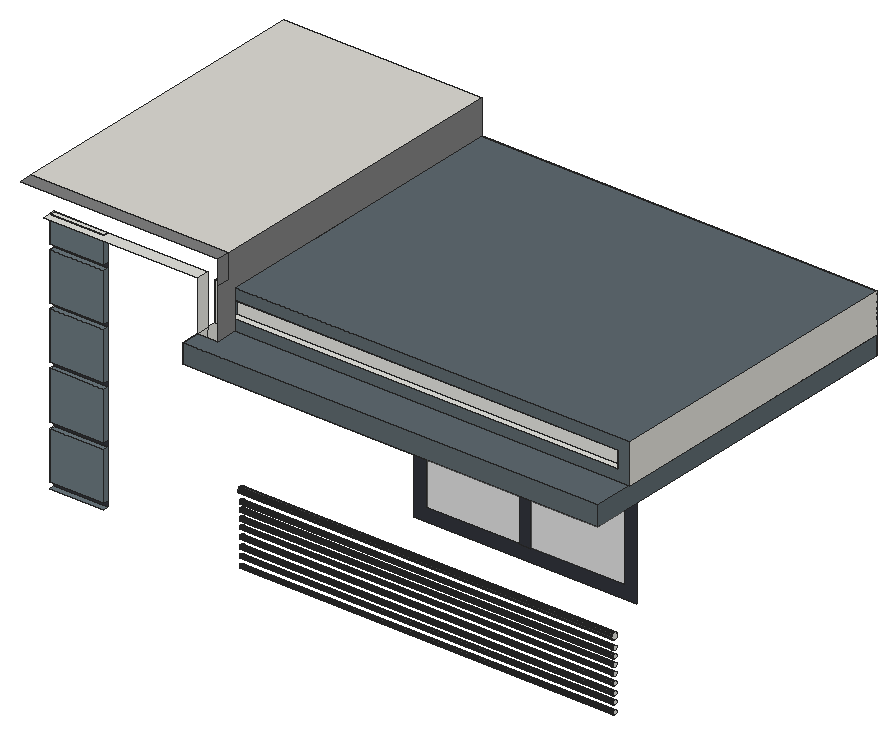
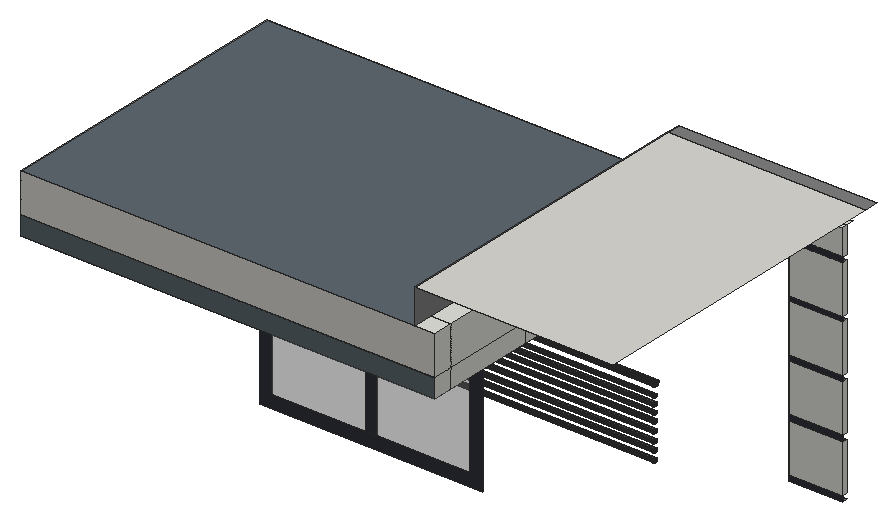
# SketchUp Ruby script. Lengths in inches.
U = 1.inch
M = Sketchup.active_model
def pt(a) = Geom::Point3d.new(a.map { |v| v * U })
def face(e, loops, mat)
  f = e.add_face(loops[0].map { |a| pt(a) })
  loops[1..].each { |l| e.add_face(l.map { |a| pt(a) }).erase! }
  f.material = f.back_material = mat if mat
  f
end
# faces: each face lists its corners as indices into pts; further lists are holes
def faces(e, pts, list, mat = nil) = list.each { |f| face(e, (f[0].is_a?(Array) ? f : [f]).map { |l| l.map { |i| pts[i] } }, mat) }
# xy, xz, yz: faces in a plane at the given z, y or x. An outline is a flat list of corners, or four numbers for a rectangle; further outlines are holes
def ring(l) = l.size == 4 ? [[l[0], l[1]], [l[2], l[1]], [l[2], l[3]], [l[0], l[3]]] : l.each_slice(2).to_a
def flat(e, list, mat, &to3) = list.each { |f| face(e, (f[0].is_a?(Array) ? f : [f]).map { |l| ring(l).map { |u, v| to3.(u, v) } }, mat) }
def xy(e, z, list, mat = nil) = flat(e, list, mat) { |x, y| [x, y, z] }
def xz(e, y, list, mat = nil) = flat(e, list, mat) { |x, z| [x, y, z] }
def yz(e, x, list, mat = nil) = flat(e, list, mat) { |y, z| [x, y, z] }
def lines(e, pts, list) = list.each { |a, b| e.add_line(pt(pts[a]), pt(pts[b])) }
# prism: a flat outline (further loops are holes) pulled along v
def prism(e, loops, v, mat = nil)
  f = face(e, loops, mat); d = Geom::Vector3d.new(v.map { |x| x * U })
  f.pushpull(f.normal.samedirection?(d) ? d.length : -d.length)
end
def box(e, o, s, mat = nil) = prism(e, [[o, [o[0] + s[0], o[1], o[2]], [o[0] + s[0], o[1] + s[1], o[2]], [o[0], o[1] + s[1], o[2]]]], [0, 0, s[2]], mat)
def at(x, y, z, deg = 0) = Geom::Transformation.translation(pt([x, y, z])) * Geom::Transformation.rotation(ORIGIN, Z_AXIS, deg.degrees)
def axes(o, x, y, z) = Geom::Transformation.new([*x, 0, *y, 0, *z, 0, *pt(o).to_a, 1])
def part(name) = M.definitions.add(name)
# library, detail: a bought-in or finely detailed component or shape, given as its bounding box
def library(name, o, s) = part(name).tap { |d| box(d.entities, o, s) }
def detail(e, o, s) = box(e.add_group.entities, o, s)
def put(e, d, t, mat = nil) = e.add_instance(d, t).tap { |i| i.material = mat if mat }
def group(e, t, mat = nil) = e.add_group.tap { |g| g.transformation = t; g.material = mat if mat }.entities
root = M.entities
M.materials.add("[0133_Gray]").color = [128, 128, 128]
M.materials.add("[Color M00]").color = [255, 255, 255]
M.materials.add("[Color M04]").color = [142, 142, 142]
M.materials.add("[Color M06]").color = [86, 86, 86]
M.materials.add("[Formica Laminate Dark]").color = [50, 53, 60]
M.materials.add("[Formica Speckled Grey]").color = [107, 120, 127]
M.materials.add("[Formica Speckled Grey]1").color = [94, 105, 111]
M.materials.add("[Terrazzo Tile Light]").color = [219, 217, 210]
M.materials.add("[Translucent Glass Gray]").color = [128, 128, 128]
M.materials["[Translucent Glass Gray]"].alpha = 0.5
xy(root,218.1875,[[22.92,75.48,40.57,77.29]],"[Formica Speckled Grey]")
xy(root,220,[[22.92,75.48,40.57,77.29]],"[Formica Speckled Grey]")
xy(root,234.625,[[169.66,81.17,169.92,81.21,170.16,81.31,170.37,81.46,170.53,81.67,170.625,81.91,170.66,82.17,170.625,82.43,170.53,82.67,170.37,82.88,170.16,83.04,169.92,83.14,169.66,83.17,169.4,83.14,169.16,83.04,168.95,82.88,168.8,82.67,168.7,82.43,168.66,82.17,168.7,81.91,168.8,81.67,168.95,81.46,169.16,81.31,169.4,81.21]])
xy(root,235,[[136.97,81.17,137.23,81.21,137.47,81.31,137.68,81.46,137.84,81.67,137.9375,81.91,137.97,82.17,137.9375,82.43,137.84,82.67,137.68,82.88,137.47,83.04,137.23,83.14,136.97,83.17,136.71,83.14,136.47,83.04,136.27,82.88,136.11,82.67,136.01,82.43,135.97,82.17,136.01,81.91,136.11,81.67,136.27,81.46,136.47,81.31,136.71,81.21]])
xy(root,235.0625,[[108.66,81.17,108.92,81.21,109.16,81.31,109.37,81.46,109.53,81.67,109.625,81.91,109.66,82.17,109.625,82.43,109.53,82.67,109.37,82.88,109.16,83.04,108.92,83.14,108.66,83.17,108.4,83.14,108.16,83.04,107.95,82.88,107.8,82.67,107.7,82.43,107.66,82.17,107.7,81.91,107.8,81.67,107.95,81.46,108.16,81.31,108.4,81.21]])
xy(root,235.75,[[22.92,75.48,40.57,77.29]],"[Formica Speckled Grey]")
xy(root,237.75,[[22.92,75.48,40.57,77.29]],"[Formica Speckled Grey]")
xy(root,253.5,[[22.92,75.48,40.57,77.29]],"[Formica Speckled Grey]")
xy(root,255.31,[[22.92,75.48,40.57,77.29]],"[Formica Speckled Grey]")
xy(root,271.0625,[[22.92,75.48,40.57,77.29]],"[Formica Speckled Grey]")
xy(root,272.68,[[22.92,75.48,40.57,77.29]],"[Formica Speckled Grey]")
xy(root,276.375,[[73.48,77.29,80.125,126.48],[202.95,77.29,209.59,126.48],[73.48,126.48,80.125,132.38],[80.125,126.48,202.95,132.38],[202.95,126.48,209.59,132.38],
  [73.48,132.38,80.125,181.19],[80.125,132.38,202.95,171.71],[202.95,132.38,209.59,181.19],[80.125,171.71,202.95,181.19]])
xy(root,276.375,[[96.82,76.93,97.66,77.05,98.44,77.37,99.11,77.89,99.63,78.56,99.96,79.34,100.07,80.18,99.96,81.03,99.63,81.81,99.11,82.48,98.44,83,97.66,83.32,96.82,83.43,95.98,83.32,95.19,83,94.52,82.48,94,81.81,93.68,81.03,93.57,80.18,93.68,79.34,94,78.56,94.52,77.89,95.19,77.37,95.98,77.05],[139.57,76.93,140.41,77.05,141.19,77.37,141.86,77.89,142.38,78.56,142.71,79.34,142.82,80.18,142.71,81.03,142.38,81.81,141.86,82.48,141.19,83,140.41,83.32,139.57,83.43,138.73,83.32,137.94,83,137.27,82.48,136.75,81.81,136.43,81.03,136.32,80.18,136.43,79.34,136.75,78.56,137.27,77.89,137.94,77.37,138.73,77.05],[177.38,76.93,178.22,77.05,179,77.37,179.68,77.89,180.19,78.56,180.52,79.34,180.63,80.18,180.52,81.03,180.19,81.81,179.68,82.48,179,83,178.22,83.32,177.38,83.43,176.54,83.32,175.75,83,175.08,82.48,174.5625,81.81,174.24,81.03,174.13,80.18,174.24,79.34,174.5625,78.56,175.08,77.89,175.75,77.37,176.54,77.05],[96.82,97.56,97.66,97.67,98.44,97.99,99.11,98.51,99.63,99.18,99.96,99.97,100.07,100.81,99.96,101.65,99.63,102.43,99.11,103.11,98.44,103.625,97.66,103.95,96.82,104.06,95.98,103.95,95.19,103.625,94.52,103.11,94,102.43,93.68,101.65,93.57,100.81,93.68,99.97,94,99.18,94.52,98.51,95.19,97.99,95.98,97.67],[143.69,97.56,144.53,97.67,145.32,97.99,145.99,98.51,146.51,99.18,146.83,99.97,146.94,100.81,146.83,101.65,146.51,102.43,145.99,103.11,145.32,103.625,144.53,103.95,143.69,104.06,142.85,103.95,142.07,103.625,141.39,103.11,140.875,102.43,140.55,101.65,140.44,100.81,140.55,99.97,140.875,99.18,141.39,98.51,142.07,97.99,142.85,97.67],
  [182,97.56,182.85,97.67,183.63,97.99,184.3,98.51,184.82,99.18,185.14,99.97,185.25,100.81,185.14,101.65,184.82,102.43,184.3,103.11,183.63,103.625,182.85,103.95,182,104.06,181.16,103.95,180.38,103.625,179.71,103.11,179.1875,102.43,178.86,101.65,178.75,100.81,178.86,99.97,179.1875,99.18,179.71,98.51,180.38,97.99,181.16,97.67]],"[Color M00]")
xy(root,276.375,[[[80.125,66.79,202.95,126.48],[96.82,76.93,95.98,77.05,95.19,77.37,94.52,77.89,94,78.56,93.68,79.34,93.57,80.18,93.68,81.03,94,81.81,94.52,82.48,95.19,83,95.98,83.32,96.82,83.43,97.66,83.32,98.44,83,99.11,82.48,99.63,81.81,99.96,81.03,100.07,80.18,99.96,79.34,99.63,78.56,99.11,77.89,98.44,77.37,97.66,77.05],[96.82,97.56,95.98,97.67,95.19,97.99,94.52,98.51,94,99.18,93.68,99.97,93.57,100.81,93.68,101.65,94,102.43,94.52,103.11,95.19,103.625,95.98,103.95,96.82,104.06,97.66,103.95,98.44,103.625,99.11,103.11,99.63,102.43,99.96,101.65,100.07,100.81,99.96,99.97,99.63,99.18,99.11,98.51,98.44,97.99,97.66,97.67],[143.69,97.56,142.85,97.67,142.07,97.99,141.39,98.51,140.875,99.18,140.55,99.97,140.44,100.81,140.55,101.65,140.875,102.43,141.39,103.11,142.07,103.625,142.85,103.95,143.69,104.06,144.53,103.95,145.32,103.625,145.99,103.11,146.51,102.43,146.83,101.65,146.94,100.81,146.83,99.97,146.51,99.18,145.99,98.51,145.32,97.99,144.53,97.67],[139.57,76.93,138.73,77.05,137.94,77.37,137.27,77.89,136.75,78.56,136.43,79.34,136.32,80.18,136.43,81.03,136.75,81.81,137.27,82.48,137.94,83,138.73,83.32,139.57,83.43,140.41,83.32,141.19,83,141.86,82.48,142.38,81.81,142.71,81.03,142.82,80.18,142.71,79.34,142.38,78.56,141.86,77.89,141.19,77.37,140.41,77.05],[182,97.56,181.16,97.67,180.38,97.99,179.71,98.51,179.1875,99.18,178.86,99.97,178.75,100.81,178.86,101.65,179.1875,102.43,179.71,103.11,180.38,103.625,181.16,103.95,182,104.06,182.85,103.95,183.63,103.625,184.3,103.11,184.82,102.43,185.14,101.65,185.25,100.81,185.14,99.97,184.82,99.18,184.3,98.51,183.63,97.99,182.85,97.67],[177.38,76.93,176.54,77.05,175.75,77.37,175.08,77.89,174.5625,78.56,174.24,79.34,174.13,80.18,174.24,81.03,174.5625,81.81,175.08,82.48,175.75,83,176.54,83.32,177.38,83.43,178.22,83.32,179,83,179.68,82.48,180.19,81.81,180.52,81.03,180.63,80.18,180.52,79.34,180.19,78.56,179.68,77.89,179,77.37,178.22,77.05]]],"[Color M04]")
xy(root,276.375,[[73.48,66.79,80.125,77.29],[202.95,66.79,209.59,77.29]],"[Formica Speckled Grey]1")
xy(root,282.625,[[73.48,79.87,209.59,181.19]])
xy(root,282.625,[[73.48,66.79,209.59,66.79,209.59,79.87,80.125,79.87,80.125,72.92,73.48,72.92]],"[Formica Speckled Grey]1")
xy(root,286.08,[[78.67,79.87,205.73,82.37]])
xy(root,288.4375,[[22.92,75.48,40.57,77.29]],"[Formica Speckled Grey]")
xy(root,290.11,[[22.92,75.48,40.57,77.29]],"[Formica Speckled Grey]")
xy(root,291.7,[[78.67,79.87,205.73,82.37]])
xy(root,295.4375,[[73.48,79.87,80.125,86.77],[73.48,86.77,80.125,113.38],[73.48,113.38,80.125,126.48],[73.48,126.48,80.125,131.65],[73.48,131.65,80.125,132.38],
  [73.48,132.38,80.125,143.96],[73.48,143.96,80.125,174.55],[73.48,174.55,80.125,181.19]])
xy(root,295.4375,[[80.125,79.87,209.59,181.19]],"[Formica Speckled Grey]1")
xy(root,298.85,[[22.92,72.92,22.92,75.48,40.57,75.48,40.57,77.29,73.48,77.29,73.48,72.92],[22.92,75.48,40.57,77.29]])
xy(root,306.8125,[[15.28,72.92,80.125,77.29]],"[0133_Gray]")
xy(root,306.8125,[[15.28,77.29,80.125,181.19]],"[Terrazzo Tile Light]")
xz(root,66.79,[[73.48,276.375,209.59,282.625]],"[Formica Speckled Grey]1")
xz(root,75.48,[[22.92,220,40.57,235.75],[22.92,237.75,40.57,253.5],[22.92,255.31,40.57,271.0625],[22.92,272.68,40.57,288.4375],[22.92,290.11,40.57,298.85]],"[Formica Speckled Grey]")
xz(root,77.29,[[22.92,220,40.57,235.75],[22.92,237.75,40.57,253.5],[22.92,255.31,40.57,271.0625],[22.92,272.68,40.57,288.4375],[22.92,290.11,40.57,298.85]])
xz(root,77.29,[[22.92,218.1875,40.57,220],[22.92,235.75,40.57,237.75],[22.92,253.5,40.57,255.31],[22.92,271.0625,40.57,272.68],[22.92,288.4375,40.57,290.11]],"[Formica Laminate Dark]")
xz(root,79.87,[[73.48,282.625,80.125,282.625,80.125,286.08,78.67,286.08,78.67,291.7,80.125,291.7,80.125,295.4375,73.48,295.4375],[78.67,286.08,80.125,291.7]])
xz(root,79.87,[[80.125,282.625,209.59,282.625,209.59,295.4375,80.125,295.4375,80.125,291.7,205.73,291.7,205.73,286.08,80.125,286.08]],"[Formica Speckled Grey]1")
xz(root,82.37,[[78.67,286.08,205.73,291.7]])
xz(root,126.48,[[[101.56,215.09,174.81,266.84],[105.7,219.23,170.66,262.69]],[136.32,219.23,140.125,262.69]],"[Formica Laminate Dark]")
xz(root,126.48,[[105.7,219.23,136.32,262.69],[140.125,219.23,170.66,262.69]],"[Translucent Glass Gray]")
xz(root,181.19,[[73.48,276.375,209.59,282.625]],"[Formica Speckled Grey]1")
xz(root,181.19,[[73.48,282.625,209.59,295.4375]],"[Terrazzo Tile Light]")
yz(root,22.92,[[75.48,220,77.29,235.75],[75.48,237.75,77.29,253.5],[75.48,255.31,77.29,271.0625],[75.48,272.68,77.29,288.4375],[75.48,290.11,77.29,298.85]])
yz(root,40.57,[[75.48,220,77.29,235.75],[75.48,237.75,77.29,253.5],[75.48,255.31,77.29,271.0625],[75.48,272.68,77.29,288.4375],[75.48,290.11,77.29,298.85]],"[Formica Speckled Grey]")
yz(root,73.48,[[66.79,276.375,77.29,282.625],[77.29,276.375,86.77,282.625],[86.77,276.375,113.38,282.625],[113.38,276.375,126.48,282.625],[126.48,276.375,131.65,282.625],
  [131.65,276.375,132.38,282.625],[132.38,276.375,143.96,282.625],[143.96,276.375,174.55,282.625],[174.55,276.375,181.19,282.625],[72.92,282.625,77.29,298.85],
  [79.87,282.625,86.77,295.4375],[86.77,282.625,113.38,295.4375],[113.38,282.625,126.48,295.4375],[126.48,282.625,131.65,295.4375],[131.65,282.625,132.38,295.4375],
  [132.38,282.625,143.96,295.4375],[143.96,282.625,174.55,295.4375],[174.55,282.625,181.19,295.4375]])
yz(root,78.67,[[79.87,286.08,82.37,291.7]],"[Formica Speckled Grey]1")
yz(root,80.125,[[72.92,282.625,79.87,282.625,79.87,295.4375,181.19,295.4375,181.19,306.8125,77.29,306.8125,77.29,298.85,72.92,298.85],[72.92,298.85,77.29,306.8125]],"[0133_Gray]")
yz(root,202.95,[[82.38,211.9,82.55,211.92,82.7,211.98,82.83,212.08,82.92,212.21,82.99,212.36,83.01,212.52,82.99,212.68,82.92,212.83,82.83,212.96,82.7,213.0625,82.55,213.125,82.38,213.15,82.22,213.125,82.07,213.0625,81.94,212.96,81.84,212.83,81.78,212.68,81.76,212.52,81.78,212.36,81.84,212.21,81.94,212.08,82.07,211.98,82.22,211.92],[82.38,214.83,82.55,214.86,82.7,214.92,82.83,215.02,82.92,215.15,82.99,215.3,83.01,215.46,82.99,215.62,82.92,215.77,82.83,215.9,82.7,216,82.55,216.0625,82.38,216.08,82.22,216.0625,82.07,216,81.94,215.9,81.84,215.77,81.78,215.62,81.76,215.46,81.78,215.3,81.84,215.15,81.94,215.02,82.07,214.92,82.22,214.86],[82.38,217.52,82.55,217.54,82.7,217.61,82.83,217.71,82.92,217.83,82.99,217.99,83.01,218.15,82.99,218.31,82.92,218.46,82.83,218.59,82.7,218.6875,82.55,218.75,82.38,218.77,82.22,218.75,82.07,218.6875,81.94,218.59,81.84,218.46,81.78,218.31,81.76,218.15,81.78,217.99,81.84,217.83,81.94,217.71,82.07,217.61,82.22,217.54],[82.38,220.46,82.55,220.48,82.7,220.54,82.83,220.64,82.92,220.77,82.99,220.92,83.01,221.08,82.99,221.25,82.92,221.4,82.83,221.53,82.7,221.625,82.55,221.6875,82.38,221.71,82.22,221.6875,82.07,221.625,81.94,221.53,81.84,221.4,81.78,221.25,81.76,221.08,81.78,220.92,81.84,220.77,81.94,220.64,82.07,220.54,82.22,220.48],[82.38,223.27,82.55,223.29,82.7,223.36,82.83,223.46,82.92,223.58,82.99,223.74,83.01,223.9,82.99,224.06,82.92,224.21,82.83,224.34,82.7,224.4375,82.55,224.5,82.38,224.52,82.22,224.5,82.07,224.4375,81.94,224.34,81.84,224.21,81.78,224.06,81.76,223.9,81.78,223.74,81.84,223.58,81.94,223.46,82.07,223.36,82.22,223.29],
  [82.38,225.9,82.55,225.92,82.7,225.98,82.83,226.08,82.92,226.21,82.99,226.36,83.01,226.52,82.99,226.68,82.92,226.83,82.83,226.96,82.7,227.0625,82.55,227.125,82.38,227.15,82.22,227.125,82.07,227.0625,81.94,226.96,81.84,226.83,81.78,226.68,81.76,226.52,81.78,226.36,81.84,226.21,81.94,226.08,82.07,225.98,82.22,225.92],[82.38,228.4,82.55,228.42,82.7,228.48,82.83,228.58,82.92,228.71,82.99,228.86,83.01,229.02,82.99,229.18,82.92,229.33,82.83,229.46,82.7,229.5625,82.55,229.625,82.38,229.65,82.22,229.625,82.07,229.5625,81.94,229.46,81.84,229.33,81.78,229.18,81.76,229.02,81.78,228.86,81.84,228.71,81.94,228.58,82.07,228.48,82.22,228.42],[82.38,230.9,82.55,230.92,82.7,230.98,82.83,231.08,82.92,231.21,82.99,231.36,83.01,231.52,82.99,231.68,82.92,231.83,82.83,231.96,82.7,232.0625,82.55,232.125,82.38,232.15,82.22,232.125,82.07,232.0625,81.94,231.96,81.84,231.83,81.78,231.68,81.76,231.52,81.78,231.36,81.84,231.21,81.94,231.08,82.07,230.98,82.22,230.92],[82.17,234.08,82.42,234.11,82.67,234.21,82.875,234.37,83.03,234.58,83.13,234.82,83.17,235.08,83.13,235.34,83.03,235.58,82.875,235.79,82.67,235.94,82.42,236.04,82.17,236.08,81.91,236.04,81.67,235.94,81.46,235.79,81.3,235.58,81.2,235.34,81.17,235.08,81.2,234.82,81.3,234.58,81.46,234.37,81.67,234.21,81.91,234.11]])
yz(root,205.73,[[79.87,286.08,82.37,291.7]],"[Formica Speckled Grey]1")
yz(root,209.59,[[66.79,276.375,181.19,282.625]],"[Formica Speckled Grey]1")
yz(root,209.59,[[79.87,282.625,181.19,295.4375]],"[Terrazzo Tile Light]")
p = [[202.95,82.22,211.92],[202.95,82.07,211.98],[80.125,82.07,211.98],[80.125,82.22,211.92],[202.95,82.38,211.9],[80.125,82.38,211.9],
  [202.95,82.55,211.92],[80.125,82.55,211.92],[202.95,82.7,211.98],[80.125,82.7,211.98],[202.95,81.94,212.08],[80.125,81.94,212.08],
  [202.95,82.83,212.08],[80.125,82.83,212.08],[202.95,81.84,212.21],[80.125,81.84,212.21],[202.95,82.92,212.21],[80.125,82.92,212.21],
  [202.95,81.78,212.36],[80.125,81.78,212.36],[202.95,82.99,212.36],[80.125,82.99,212.36],[202.95,81.76,212.52],[80.125,81.76,212.52],
  [202.95,83.01,212.52],[80.125,83.01,212.52],[202.95,81.78,212.68],[80.125,81.78,212.68],[202.95,82.99,212.68],[80.125,82.99,212.68],
  [202.95,81.84,212.83],[80.125,81.84,212.83],[202.95,82.92,212.83],[80.125,82.92,212.83],[202.95,81.94,212.96],[80.125,81.94,212.96],
  [202.95,82.83,212.96],[80.125,82.83,212.96],[202.95,82.07,213.0625],[80.125,82.07,213.0625],[202.95,82.7,213.0625],[80.125,82.7,213.0625],
  [202.95,82.22,213.125],[80.125,82.22,213.125],[202.95,82.38,213.15],[80.125,82.38,213.15],[202.95,82.55,213.125],[80.125,82.55,213.125],
  [202.95,82.38,214.83],[202.95,82.22,214.86],[80.125,82.22,214.86],[80.125,82.38,214.83],[202.95,82.55,214.86],[80.125,82.55,214.86],
  [202.95,82.07,214.92],[202.95,81.94,215.02],[80.125,81.94,215.02],[80.125,82.07,214.92],[202.95,82.7,214.92],[80.125,82.7,214.92],
  [202.95,82.83,215.02],[80.125,82.83,215.02],[202.95,81.84,215.15],[80.125,81.84,215.15],[202.95,82.92,215.15],[80.125,82.92,215.15],
  [202.95,81.78,215.3],[80.125,81.78,215.3],[202.95,82.99,215.3],[80.125,82.99,215.3],[202.95,81.76,215.46],[80.125,81.76,215.46],
  [202.95,83.01,215.46],[80.125,83.01,215.46],[202.95,81.78,215.62],[80.125,81.78,215.62],[202.95,82.99,215.62],[80.125,82.99,215.62],
  [202.95,81.84,215.77],[80.125,81.84,215.77],[202.95,82.92,215.77],[80.125,82.92,215.77],[202.95,81.94,215.9],[80.125,81.94,215.9],
  [202.95,82.83,215.9],[80.125,82.83,215.9],[202.95,82.07,216],[80.125,82.07,216],[202.95,82.7,216],[80.125,82.7,216],
  [202.95,82.22,216.0625],[80.125,82.22,216.0625],[202.95,82.55,216.0625],[80.125,82.55,216.0625],[202.95,82.38,216.08],[80.125,82.38,216.08],
  [202.95,82.22,217.54],[202.95,82.07,217.61],[80.125,82.07,217.61],[80.125,82.22,217.54],[202.95,82.38,217.52],[80.125,82.38,217.52],
  [202.95,82.55,217.54],[80.125,82.55,217.54],[202.95,82.7,217.61],[80.125,82.7,217.61],[202.95,81.94,217.71],[80.125,81.94,217.71],
  [202.95,82.83,217.71],[80.125,82.83,217.71],[202.95,81.84,217.83],[80.125,81.84,217.83],[202.95,82.92,217.83],[80.125,82.92,217.83],
  [202.95,81.78,217.99],[80.125,81.78,217.99],[202.95,82.99,217.99],[80.125,82.99,217.99],[202.95,81.76,218.15],[80.125,81.76,218.15],
  [202.95,83.01,218.15],[80.125,83.01,218.15],[202.95,81.78,218.31],[80.125,81.78,218.31],[202.95,82.99,218.31],[80.125,82.99,218.31],
  [202.95,81.84,218.46],[80.125,81.84,218.46],[202.95,82.92,218.46],[80.125,82.92,218.46],[202.95,81.94,218.59],[80.125,81.94,218.59],
  [202.95,82.83,218.59],[80.125,82.83,218.59],[202.95,82.07,218.6875],[80.125,82.07,218.6875],[202.95,82.7,218.6875],[80.125,82.7,218.6875],
  [202.95,82.22,218.75],[80.125,82.22,218.75],[202.95,82.55,218.75],[80.125,82.55,218.75],[202.95,82.38,218.77],[80.125,82.38,218.77],
  [202.95,82.07,220.54],[202.95,81.94,220.64],[80.125,81.94,220.64],[80.125,82.07,220.54],[202.95,82.22,220.48],[80.125,82.22,220.48],
  [202.95,82.38,220.46],[80.125,82.38,220.46],[202.95,82.55,220.48],[80.125,82.55,220.48],[202.95,82.7,220.54],[80.125,82.7,220.54],
  [202.95,82.83,220.64],[80.125,82.83,220.64],[202.95,81.84,220.77],[80.125,81.84,220.77],[202.95,82.92,220.77],[80.125,82.92,220.77],
  [202.95,81.78,220.92],[80.125,81.78,220.92],[202.95,82.99,220.92],[80.125,82.99,220.92],[202.95,81.76,221.08],[80.125,81.76,221.08],
  [202.95,83.01,221.08],[80.125,83.01,221.08],[202.95,81.78,221.25],[80.125,81.78,221.25],[202.95,82.99,221.25],[80.125,82.99,221.25],
  [202.95,81.84,221.4],[80.125,81.84,221.4],[202.95,82.92,221.4],[80.125,82.92,221.4],[202.95,81.94,221.53],[80.125,81.94,221.53],
  [202.95,82.83,221.53],[80.125,82.83,221.53],[202.95,82.07,221.625],[80.125,82.07,221.625],[202.95,82.7,221.625],[80.125,82.7,221.625],
  [202.95,82.22,221.6875],[80.125,82.22,221.6875],[202.95,82.55,221.6875],[80.125,82.55,221.6875],[202.95,82.38,221.71],[80.125,82.38,221.71],
  [202.95,82.22,223.29],[202.95,82.07,223.36],[80.125,82.07,223.36],[80.125,82.22,223.29],[202.95,82.38,223.27],[80.125,82.38,223.27],
  [202.95,82.55,223.29],[80.125,82.55,223.29],[202.95,82.7,223.36],[80.125,82.7,223.36],[202.95,81.94,223.46],[80.125,81.94,223.46],
  [202.95,82.83,223.46],[80.125,82.83,223.46],[202.95,81.84,223.58],[80.125,81.84,223.58],[202.95,82.92,223.58],[80.125,82.92,223.58],
  [202.95,81.78,223.74],[80.125,81.78,223.74],[202.95,82.99,223.74],[80.125,82.99,223.74],[202.95,81.76,223.9],[80.125,81.76,223.9],
  [202.95,83.01,223.9],[80.125,83.01,223.9],[202.95,81.78,224.06],[80.125,81.78,224.06],[202.95,82.99,224.06],[80.125,82.99,224.06],
  [202.95,81.84,224.21],[80.125,81.84,224.21],[202.95,82.92,224.21],[80.125,82.92,224.21],[202.95,81.94,224.34],[80.125,81.94,224.34],
  [202.95,82.83,224.34],[80.125,82.83,224.34],[202.95,82.07,224.4375],[80.125,82.07,224.4375],[202.95,82.7,224.4375],[80.125,82.7,224.4375],
  [202.95,82.22,224.5],[80.125,82.22,224.5],[202.95,82.55,224.5],[80.125,82.55,224.5],[202.95,82.38,224.52],[80.125,82.38,224.52],
  [202.95,82.22,225.92],[202.95,82.07,225.98],[80.125,82.07,225.98],[80.125,82.22,225.92],[202.95,82.38,225.9],[80.125,82.38,225.9],
  [202.95,82.55,225.92],[80.125,82.55,225.92],[202.95,82.7,225.98],[80.125,82.7,225.98],[202.95,81.94,226.08],[80.125,81.94,226.08],
  [202.95,82.83,226.08],[80.125,82.83,226.08],[202.95,81.84,226.21],[80.125,81.84,226.21],[202.95,82.92,226.21],[80.125,82.92,226.21],
  [202.95,81.78,226.36],[80.125,81.78,226.36],[202.95,82.99,226.36],[80.125,82.99,226.36],[202.95,81.76,226.52],[80.125,81.76,226.52],
  [202.95,83.01,226.52],[80.125,83.01,226.52],[202.95,81.78,226.68],[80.125,81.78,226.68],[202.95,82.99,226.68],[80.125,82.99,226.68],
  [202.95,81.84,226.83],[80.125,81.84,226.83],[202.95,82.92,226.83],[80.125,82.92,226.83],[202.95,81.94,226.96],[80.125,81.94,226.96],
  [202.95,82.83,226.96],[80.125,82.83,226.96],[202.95,82.07,227.0625],[80.125,82.07,227.0625],[202.95,82.7,227.0625],[80.125,82.7,227.0625],
  [202.95,82.22,227.125],[80.125,82.22,227.125],[202.95,82.38,227.15],[80.125,82.38,227.15],[202.95,82.55,227.125],[80.125,82.55,227.125],
  [202.95,82.22,228.42],[202.95,82.07,228.48],[80.125,82.07,228.48],[80.125,82.22,228.42],[202.95,82.38,228.4],[80.125,82.38,228.4],
  [202.95,82.55,228.42],[80.125,82.55,228.42],[202.95,82.7,228.48],[80.125,82.7,228.48],[202.95,81.94,228.58],[80.125,81.94,228.58],
  [202.95,82.83,228.58],[80.125,82.83,228.58],[202.95,81.84,228.71],[80.125,81.84,228.71],[202.95,82.92,228.71],[80.125,82.92,228.71],
  [202.95,81.78,228.86],[80.125,81.78,228.86],[202.95,82.99,228.86],[80.125,82.99,228.86],[202.95,81.76,229.02],[80.125,81.76,229.02],
  [202.95,83.01,229.02],[80.125,83.01,229.02],[202.95,81.78,229.18],[80.125,81.78,229.18],[202.95,82.99,229.18],[80.125,82.99,229.18],
  [202.95,81.84,229.33],[80.125,81.84,229.33],[202.95,82.92,229.33],[80.125,82.92,229.33],[202.95,81.94,229.46],[80.125,81.94,229.46],
  [202.95,82.83,229.46],[80.125,82.83,229.46],[202.95,82.07,229.5625],[80.125,82.07,229.5625],[202.95,82.7,229.5625],[80.125,82.7,229.5625],
  [202.95,82.22,229.625],[80.125,82.22,229.625],[202.95,82.38,229.65],[80.125,82.38,229.65],[202.95,82.55,229.625],[80.125,82.55,229.625],
  [202.95,82.22,230.92],[202.95,82.07,230.98],[80.125,82.07,230.98],[80.125,82.22,230.92],[202.95,82.38,230.9],[80.125,82.38,230.9],
  [202.95,82.55,230.92],[80.125,82.55,230.92],[202.95,82.7,230.98],[80.125,82.7,230.98],[202.95,81.94,231.08],[80.125,81.94,231.08],
  [202.95,82.83,231.08],[80.125,82.83,231.08],[202.95,81.84,231.21],[80.125,81.84,231.21],[202.95,82.92,231.21],[80.125,82.92,231.21],
  [202.95,81.78,231.36],[80.125,81.78,231.36],[202.95,82.99,231.36],[80.125,82.99,231.36],[202.95,81.76,231.52],[80.125,81.76,231.52],
  [202.95,83.01,231.52],[80.125,83.01,231.52],[202.95,81.78,231.68],[80.125,81.78,231.68],[202.95,82.99,231.68],[80.125,82.99,231.68],
  [202.95,81.84,231.83],[80.125,81.84,231.83],[202.95,82.92,231.83],[80.125,82.92,231.83],[202.95,81.94,231.96],[80.125,81.94,231.96],
  [202.95,82.83,231.96],[80.125,82.83,231.96],[202.95,82.07,232.0625],[80.125,82.07,232.0625],[202.95,82.7,232.0625],[80.125,82.7,232.0625],
  [202.95,82.22,232.125],[80.125,82.22,232.125],[202.95,82.38,232.15],[80.125,82.38,232.15],[202.95,82.55,232.125],[80.125,82.55,232.125],
  [202.95,81.91,234.11],[202.95,81.67,234.21],[80.125,81.67,234.21],[80.125,81.91,234.11],[202.95,82.17,234.08],[80.125,82.17,234.08],
  [202.95,82.42,234.11],[80.125,82.42,234.11],[202.95,82.67,234.21],[80.125,82.67,234.21],[202.95,81.46,234.37],[80.125,81.46,234.37],
  [202.95,82.875,234.37],[80.125,82.875,234.37],[202.95,81.3,234.58],[80.125,81.3,234.58],[202.95,83.03,234.58],[80.125,83.03,234.58],
  [202.95,81.2,234.82],[80.125,81.2,234.82],[202.95,83.13,234.82],[80.125,83.13,234.82],[202.95,81.17,235.08],[80.125,81.17,235.08],
  [202.95,83.17,235.08],[80.125,83.17,235.08],[202.95,81.2,235.34],[80.125,81.2,235.34],[202.95,83.13,235.34],[80.125,83.13,235.34],
  [202.95,81.3,235.58],[80.125,81.3,235.58],[202.95,83.03,235.58],[80.125,83.03,235.58],[202.95,81.46,235.79],[80.125,81.46,235.79],
  [202.95,82.875,235.79],[80.125,82.875,235.79],[202.95,81.67,235.94],[80.125,81.67,235.94],[202.95,82.67,235.94],[80.125,82.67,235.94],
  [202.95,81.91,236.04],[80.125,81.91,236.04],[202.95,82.42,236.04],[80.125,82.42,236.04],[202.95,82.17,236.08],[80.125,82.17,236.08]]
faces(root,p,[[0,1,2,3],[4,0,3,5],[6,4,5,7],[8,6,7,9],[1,10,11,2],[12,8,9,13],[10,14,15,11],[16,12,13,17],
  [14,18,19,15],[20,16,17,21],[18,22,23,19],[24,20,21,25],[22,26,27,23],[28,24,25,29],[26,30,31,27],[32,28,29,33],
  [30,34,35,31],[36,32,33,37],[34,38,39,35],[40,36,37,41],[38,42,43,39],[42,44,45,43],[44,46,47,45],[46,40,41,47],
  [48,49,50,51],[52,48,51,53],[54,55,56,57],[49,54,57,50],[58,52,53,59],[60,58,59,61],[55,62,63,56],[64,60,61,65],
  [62,66,67,63],[68,64,65,69],[66,70,71,67],[72,68,69,73],[70,74,75,71],[76,72,73,77],[74,78,79,75],[80,76,77,81],
  [78,82,83,79],[84,80,81,85],[82,86,87,83],[88,84,85,89],[86,90,91,87],[92,88,89,93],[90,94,95,91],[94,92,93,95],
  [96,97,98,99],[100,96,99,101],[102,100,101,103],[104,102,103,105],[97,106,107,98],[108,104,105,109],[106,110,111,107],[112,108,109,113],
  [110,114,115,111],[116,112,113,117],[114,118,119,115],[120,116,117,121],[118,122,123,119],[124,120,121,125],[122,126,127,123],[128,124,125,129],
  [126,130,131,127],[132,128,129,133],[130,134,135,131],[136,132,133,137],[134,138,139,135],[140,136,137,141],[138,142,143,139],[142,140,141,143],
  [144,145,146,147],[148,144,147,149],[150,148,149,151],[152,150,151,153],[154,152,153,155],[156,154,155,157],[145,158,159,146],[160,156,157,161],
  [158,162,163,159],[164,160,161,165],[162,166,167,163],[168,164,165,169],[166,170,171,167],[172,168,169,173],[170,174,175,171],[176,172,173,177],
  [174,178,179,175],[180,176,177,181],[178,182,183,179],[184,180,181,185],[182,186,187,183],[188,184,185,189],[186,190,191,187],[190,188,189,191],
  [192,193,194,195],[196,192,195,197],[198,196,197,199],[200,198,199,201],[193,202,203,194],[204,200,201,205],[202,206,207,203],[208,204,205,209],
  [206,210,211,207],[212,208,209,213],[210,214,215,211],[216,212,213,217],[214,218,219,215],[220,216,217,221],[218,222,223,219],[224,220,221,225],
  [222,226,227,223],[228,224,225,229],[226,230,231,227],[232,228,229,233],[230,234,235,231],[236,232,233,237],[234,238,239,235],[238,236,237,239],
  [240,241,242,243],[244,240,243,245],[246,244,245,247],[248,246,247,249],[241,250,251,242],[252,248,249,253],[250,254,255,251],[256,252,253,257],
  [254,258,259,255],[260,256,257,261],[258,262,263,259],[264,260,261,265],[262,266,267,263],[268,264,265,269],[266,270,271,267],[272,268,269,273],
  [270,274,275,271],[276,272,273,277],[274,278,279,275],[280,276,277,281],[278,282,283,279],[282,284,285,283],[284,286,287,285],[286,280,281,287],
  [288,289,290,291],[292,288,291,293],[294,292,293,295],[296,294,295,297],[289,298,299,290],[300,296,297,301],[298,302,303,299],[304,300,301,305],
  [302,306,307,303],[308,304,305,309],[306,310,311,307],[312,308,309,313],[310,314,315,311],[316,312,313,317],[314,318,319,315],[320,316,317,321],
  [318,322,323,319],[324,320,321,325],[322,326,327,323],[328,324,325,329],[326,330,331,327],[330,332,333,331],[332,334,335,333],[334,328,329,335],
  [336,337,338,339],[340,336,339,341],[342,340,341,343],[344,342,343,345],[337,346,347,338],[348,344,345,349],[346,350,351,347],[352,348,349,353],
  [350,354,355,351],[356,352,353,357],[354,358,359,355],[360,356,357,361],[358,362,363,359],[364,360,361,365],[362,366,367,363],[368,364,365,369],
  [366,370,371,367],[372,368,369,373],[370,374,375,371],[376,372,373,377],[374,378,379,375],[378,380,381,379],[380,382,383,381],[382,376,377,383],
  [384,385,386,387],[388,384,387,389],[390,388,389,391],[392,390,391,393],[385,394,395,386],[396,392,393,397],[394,398,399,395],[400,396,397,401],
  [398,402,403,399],[404,400,401,405],[402,406,407,403],[408,404,405,409],[406,410,411,407],[412,408,409,413],[410,414,415,411],[416,412,413,417],
  [414,418,419,415],[420,416,417,421],[418,422,423,419],[424,420,421,425],[422,426,427,423],[428,424,425,429],[426,430,431,427],[430,428,429,431]],"[Color M06]")
